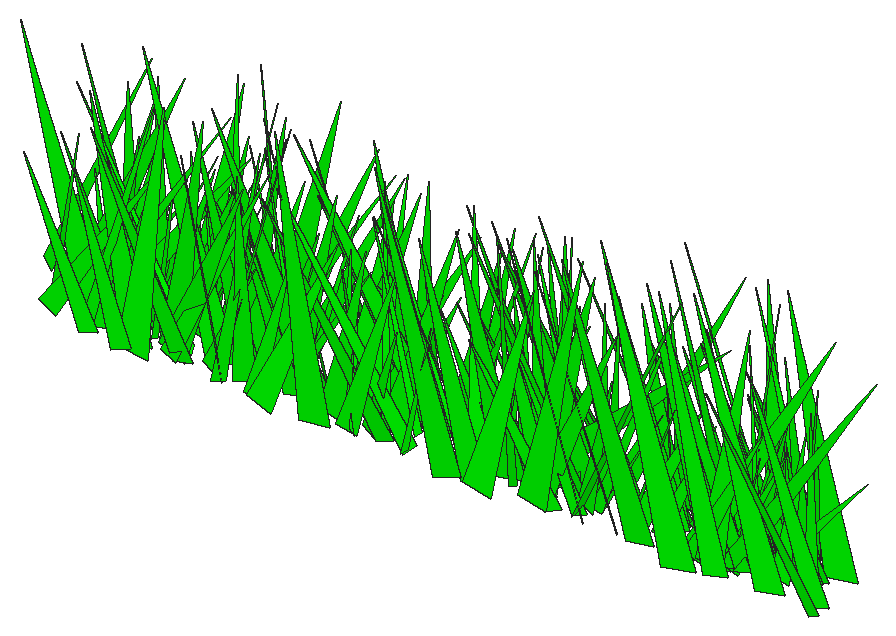
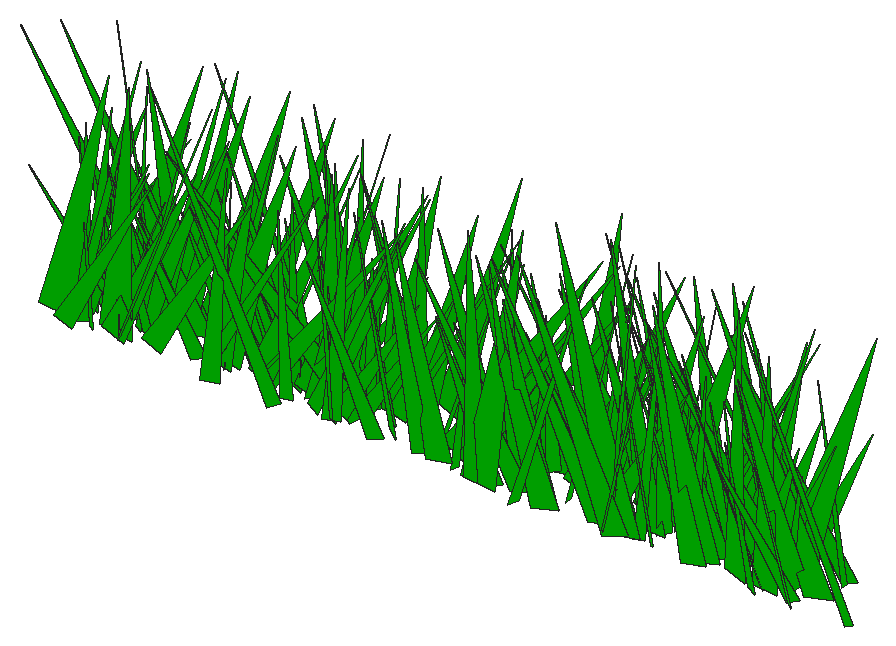
# SketchUp Ruby script. Lengths in inches.
U = 1.inch
M = Sketchup.active_model
def pt(a) = Geom::Point3d.new(a.map { |v| v * U })
def face(e, loops, mat)
  f = e.add_face(loops[0].map { |a| pt(a) })
  loops[1..].each { |l| e.add_face(l.map { |a| pt(a) }).erase! }
  f.material = f.back_material = mat if mat
  f
end
# faces: each face lists its corners as indices into pts; further lists are holes
def faces(e, pts, list, mat = nil) = list.each { |f| face(e, (f[0].is_a?(Array) ? f : [f]).map { |l| l.map { |i| pts[i] } }, mat) }
# xy, xz, yz: faces in a plane at the given z, y or x. An outline is a flat list of corners, or four numbers for a rectangle; further outlines are holes
def ring(l) = l.size == 4 ? [[l[0], l[1]], [l[2], l[1]], [l[2], l[3]], [l[0], l[3]]] : l.each_slice(2).to_a
def flat(e, list, mat, &to3) = list.each { |f| face(e, (f[0].is_a?(Array) ? f : [f]).map { |l| ring(l).map { |u, v| to3.(u, v) } }, mat) }
def xy(e, z, list, mat = nil) = flat(e, list, mat) { |x, y| [x, y, z] }
def xz(e, y, list, mat = nil) = flat(e, list, mat) { |x, z| [x, y, z] }
def yz(e, x, list, mat = nil) = flat(e, list, mat) { |y, z| [x, y, z] }
def lines(e, pts, list) = list.each { |a, b| e.add_line(pt(pts[a]), pt(pts[b])) }
# prism: a flat outline (further loops are holes) pulled along v
def prism(e, loops, v, mat = nil)
  f = face(e, loops, mat); d = Geom::Vector3d.new(v.map { |x| x * U })
  f.pushpull(f.normal.samedirection?(d) ? d.length : -d.length)
end
def box(e, o, s, mat = nil) = prism(e, [[o, [o[0] + s[0], o[1], o[2]], [o[0] + s[0], o[1] + s[1], o[2]], [o[0], o[1] + s[1], o[2]]]], [0, 0, s[2]], mat)
def at(x, y, z, deg = 0) = Geom::Transformation.translation(pt([x, y, z])) * Geom::Transformation.rotation(ORIGIN, Z_AXIS, deg.degrees)
def axes(o, x, y, z) = Geom::Transformation.new([*x, 0, *y, 0, *z, 0, *pt(o).to_a, 1])
def part(name) = M.definitions.add(name)
# library, detail: a bought-in or finely detailed component or shape, given as its bounding box
def library(name, o, s) = part(name).tap { |d| box(d.entities, o, s) }
def detail(e, o, s) = box(e.add_group.entities, o, s)
def put(e, d, t, mat = nil) = e.add_instance(d, t).tap { |i| i.material = mat if mat }
def group(e, t, mat = nil) = e.add_group.tap { |g| g.transformation = t; g.material = mat if mat }.entities
root = M.entities
M.materials.add("[0065_Lime]").color = [0, 255, 0]
c1 = part("fur_instance\#9")
p = [[0.8125,0,1.79],[0.67,-0.02,1.48],[0,-0.11,0],[0,0.11,0]]
faces(c1.entities,p,[[0,1,2,3]])
put(root,c1,axes([102.21,26.05,1.48],[1.7547,1.16122,2.32218],[-8.46058,0.32869,-1.27782],[-2.20466,-0.33717,6.75196]),"[0065_Lime]")
put(root,c1,axes([123.31,25.84,1.48],[-1.5424,1.29726,0.5634],[-9.04708,-0.19027,-1.70729],[-1.96466,-0.14229,7.41961]),"[0065_Lime]")
put(root,c1,axes([111.69,25.86,1.48],[-1.10332,1.04471,0.27422],[-7.18185,-0.16201,1.56413],[1.95185,-0.00559,5.91025]),"[0065_Lime]")
put(root,c1,axes([109.89,25.96,1.48],[3.37414,1.16063,2.27988],[-7.67588,0.59567,-2.64497],[-4.14231,-0.15841,6.75834]),"[0065_Lime]")
put(root,c1,axes([106.98,26.59,1.48],[4.6883,-0.22426,0.48877],[1.33627,0.63657,1.30663],[-1.05954,-0.18951,3.81064]),"[0065_Lime]")
put(root,c1,axes([91.18,25.96,1.48],[1.11734,0.80378,0.05922],[-5.21364,0.14737,-1.94062],[-2.35444,0.05511,4.32539]),"[0065_Lime]")
put(root,c1,axes([99.17,25.87,1.48],[-1.68486,0.94414,0.02379],[-6.07569,-0.21589,2.40069],[2.86921,0.09727,5.09755]),"[0065_Lime]")
put(root,c1,axes([91.78,26.04,1.48],[-1.91905,1.11623,1.28489],[-7.93462,-0.30486,1.0337],[1.62457,-0.17042,6.56651]),"[0065_Lime]")
put(root,c1,axes([98.54,26.24,1.48],[-1.07859,0.61607,1.11572],[-4.32863,-0.20259,0.97977],[1.53823,-0.13812,3.53945]),"[0065_Lime]")
put(root,c1,axes([130.69,26.3125,1.48],[-5.79002,-0.44025,0.10676],[3.0058,-0.76816,1.71372],[-0.89348,0.26874,5.07335]),"[0065_Lime]")
put(root,c1,axes([124.97,26.41,1.48],[-6.3055,0.74654,2.04882],[-5.78447,-0.88065,-1.02622],[1.05354,-0.36713,6.62786]),"[0065_Lime]")
put(root,c1,axes([89.08,26.29,1.48],[-2.14765,0.68234,0.54136],[-4.74981,-0.26455,-1.29382],[-1.20923,-0.17271,4.12059]),"[0065_Lime]")
put(root,c1,axes([114.36,26.49,1.48],[3.62527,0.99891,2.4784],[-7.73426,0.46872,1.15493],[-0.00819,-0.47235,6.38732]),"[0065_Lime]")
put(root,c1,axes([96.35,26.7,1.48],[-6.74477,-0.19585,1.4121],[1.05256,-0.96631,-1.16464],[1.96177,-0.1549,5.4798]),"[0065_Lime]")
put(root,c1,axes([111.2,26.3,1.48],[0.41444,0.99584,1.54491],[-7.02435,0.13106,-1.58405],[-2.11909,-0.23967,5.55294]),"[0065_Lime]")
put(root,c1,axes([103.67,26.52,1.48],[2.05749,-0.71511,1.47796],[5.3628,0.23665,-1.10273],[0.66397,0.30458,4.32675]),"[0065_Lime]")
put(root,c1,axes([116.95,26.78,1.48],[-8.41983,-0.27343,1.12929],[1.68169,-1.18523,-1.32039],[1.6988,-0.18194,6.9042]),"[0065_Lime]")
put(root,c1,axes([120.48,26.59,1.48],[-3.81513,-1.0233,1.83212],[7.58861,-0.4764,1.53917],[-0.72074,0.40077,6.5077]),"[0065_Lime]")
put(root,c1,axes([107.1,26.82,1.48],[-7.50723,0.41992,0.59815],[-3.0118,-0.94646,-2.74542],[-0.63269,-0.47719,5.97164]),"[0065_Lime]")
put(root,c1,axes([115.54,26.54,1.48],[-2.49387,0.61789,0.35428],[-4.10879,-0.29841,-1.697],[-1.62573,-0.19365,3.74544]),"[0065_Lime]")
put(root,c1,axes([104.59,27.01,1.48],[-2.3394,-0.59166,0.20628],[3.54462,-0.29782,-2.02693],[2.28668,-0.14364,3.35302]),"[0065_Lime]")
put(root,c1,axes([116.53,27.02,1.48],[9.28519,-0.22692,0.14299],[1.53138,1.27057,1.77261],[-0.54197,-0.29762,7.45832]),"[0065_Lime]")
put(root,c1,axes([94.07,26.78,1.48],[-4.00819,-0.79191,0.76199],[5.61604,-0.51668,1.55272],[-1.04793,0.25999,5.40673]),"[0065_Lime]")
put(root,c1,axes([93.17,27.14,1.48],[-1.34104,-1.06333,0.3975],[6.82997,-0.19967,-2.65233],[3.29441,-0.01889,5.6606]),"[0065_Lime]")
put(root,c1,axes([105.66,26.82,1.48],[-4.89101,-0.7549,0.09144],[5.11683,-0.64778,1.88363],[-1.64083,0.23016,5.60141]),"[0065_Lime]")
put(root,c1,axes([119.13,26.63,1.48],[-7.69959,-0.10862,0.71828],[0.9253,-1.0684,1.14867],[0.72189,0.21091,6.18874]),"[0065_Lime]")
put(root,c1,axes([111.54,26.7,1.48],[-7.68571,-0.19114,0.0547],[1.35022,-1.06232,1.1351],[-0.17805,0.19472,6.24652]),"[0065_Lime]")
put(root,c1,axes([114.32,27.02,1.48],[3.75349,-0.83573,0.21049],[5.86726,0.51206,-1.09875],[1.00756,0.13155,5.61414]),"[0065_Lime]")
put(root,c1,axes([97.33,27.16,1.48],[4.32558,-0.81356,0.76166],[5.55616,0.62078,1.34166],[-1.87806,-0.03725,5.72352]),"[0065_Lime]")
put(root,c1,axes([104.02,26.51,1.48],[4.22809,0.04304,1.71651],[0.74399,0.58735,-1.70596],[-1.99837,0.30972,2.99662]),"[0065_Lime]")
put(root,c1,axes([88.56,26.74,1.48],[7.61975,-0.23734,1.45771],[2.02283,1.07025,-1.15684],[-1.40453,0.25377,6.24217]),"[0065_Lime]")
put(root,c1,axes([93.22,26.82,1.48],[5.99973,0.64849,0.4783],[-4.63193,0.82003,1.18719],[0.43521,-0.21248,6.04147]),"[0065_Lime]")
put(root,c1,axes([127.85,26.72,1.48],[2.99159,-0.87631,4.59081],[7.42678,0.67032,1.08546],[-3.94812,0.59694,5.52044]),"[0065_Lime]")
put(root,c1,axes([114.21,27.2,1.48],[3.02124,-1.08196,0.95783],[7.76367,0.40389,-0.91484],[0.63141,0.21091,6.66551]),"[0065_Lime]")
put(root,c1,axes([102.27,27.125,1.48],[-0.14869,-0.83482,1.14694],[5.953,-0.06392,-1.04827],[1.35853,0.1887,4.71898]),"[0065_Lime]")
put(root,c1,axes([86.19,26.92,1.48],[4.36671,0.71514,0.39873],[-4.84361,0.54959,2.0661],[1.63745,-0.28142,5.04826]),"[0065_Lime]")
put(root,c1,axes([91.52,26.67,1.48],[-1.20291,1.07757,0.71265],[-7.6214,-0.14613,-1.10764],[-1.22014,-0.14958,6.21607]),"[0065_Lime]")
put(root,c1,axes([96.39,26.48,1.48],[6.48375,0.70369,0.55989],[-4.60974,0.88766,-2.06362],[-2.07422,0.22691,6.33633]),"[0065_Lime]")
put(root,c1,axes([130.41,26.98,1.48],[-4.31695,0.71055,1.29643],[-5.29641,-0.56479,-1.29621],[-0.24161,-0.31487,5.25057]),"[0065_Lime]")
put(root,c1,axes([116.68,26.99,1.48],[-3.03929,0.52441,0.66866],[-3.75819,-0.38343,-1.22573],[-0.69236,-0.22071,3.71813]),"[0065_Lime]")
put(root,c1,axes([86.16,27.32,1.48],[5.92393,0.15481,1.78214],[-1.86022,0.80815,1.7389],[-1.59798,-0.36688,4.58238]),"[0065_Lime]")
put(root,c1,axes([112.17,27.6,1.48],[1.49735,-1.20236,0.06671],[8.3405,0.20769,1.56803],[-1.91273,-0.03563,6.88965]),"[0065_Lime]")
put(root,c1,axes([123.05,27.09,1.48],[2.02452,-0.64693,1.18017],[4.62597,0.19687,-1.63434],[1.37886,0.28937,3.75031]),"[0065_Lime]")
put(root,c1,axes([96.22,26.6,1.48],[8.82311,0.3951,1.03383],[-2.25651,1.19516,-2.5638],[-2.10468,0.37495,7.08272]),"[0065_Lime]")
put(root,c1,axes([95.14,27.22,1.48],[3.25571,0.32358,0.89348],[-2.54741,0.39839,1.30694],[0.14161,-0.27277,2.96877]),"[0065_Lime]")
put(root,c1,axes([119.39,26.97,1.48],[5.10806,0.03443,0.5675],[-0.08817,0.70776,-0.91388],[-0.73419,0.15457,4.05811]),"[0065_Lime]")
put(root,c1,axes([124.47,27.18,1.48],[-2.0294,1.06878,2.47195],[-8.07706,-0.18812,-1.66187],[-1.35942,-0.47779,6.18385]),"[0065_Lime]")
put(root,c1,axes([125.18,27.48,1.48],[4.46412,-0.18338,0.40179],[1.0179,0.58709,1.49617],[-0.95449,-0.23159,3.47473]),"[0065_Lime]")
put(root,c1,axes([124.1,27.05,1.48],[4.86592,-0.74135,2.94554],[6.30982,0.66225,-1.31143],[-1.06488,0.53652,5.6888]),"[0065_Lime]")
put(root,c1,axes([92.95,27.55,1.48],[-2.67145,-1.06307,1.53834],[7.41878,-0.43302,-1.50304],[2.40291,0.15503,6.35076]),"[0065_Lime]")
put(root,c1,axes([89.19,26.93,1.48],[-1.2719,1.30197,0.61878],[-9.00315,-0.1456,-1.9784],[-2.31768,-0.14889,7.34561]),"[0065_Lime]")
put(root,c1,axes([126.86,27.16,1.48],[-6.89711,0.19534,2.04472],[-1.04841,-1.02654,0.94629],[2.67436,0.10134,5.64424]),"[0065_Lime]")
put(root,c1,axes([99.89,27.5,1.48],[-0.65863,-0.72216,0.74708],[5.05605,-0.05582,1.14126],[-1.30097,0.14868,4.05712]),"[0065_Lime]")
put(root,c1,axes([114.41,27.92,1.48],[7.30262,-0.46788,0.93542],[2.47118,0.94547,3.08221],[-2.51048,-0.43032,5.75496]),"[0065_Lime]")
put(root,c1,axes([103.85,27.76,1.48],[-4.5948,-0.46783,0.32278],[2.92083,-0.60494,-1.87066],[1.64644,-0.23241,4.2194]),"[0065_Lime]")
put(root,c1,axes([116.51,27.64,1.48],[-2.36556,-0.63281,0.7363],[4.04229,-0.35473,-1.6233],[2.1817,-0.02888,3.80603]),"[0065_Lime]")
put(root,c1,axes([124.99,27.3,1.48],[7.74588,-0.59537,0.16584],[4.07919,1.02912,-2.25937],[1.16355,0.35557,6.81694]),"[0065_Lime]")
put(root,c1,axes([112.71,27.1875,1.48],[-6.89012,-0.28564,2.5667],[2.88207,-0.99639,1.4033],[2.40473,0.37575,5.67232]),"[0065_Lime]")
put(root,c1,axes([125.5,27.34,1.48],[-0.53049,0.95921,1.54038],[-6.75326,0.01211,-1.79154],[-2.1394,-0.27608,5.27326]),"[0065_Lime]")
put(root,c1,axes([122.91,27.48,1.48],[6.46797,0.95534,0.6255],[-6.66624,0.84641,2.29021],[1.54112,-0.34829,7.28128]),"[0065_Lime]")
put(root,c1,axes([93.75,27.89,1.48],[-8.32403,-0.05832,0.19902],[0.34032,-1.13292,-1.70662],[0.34102,-0.29292,6.56096]),"[0065_Lime]")
put(root,c1,axes([89.32,27.81,1.48],[-2.17451,-0.51292,1.01396],[3.23893,-0.352,-1.37089],[2.09456,0.01183,3.17253]),"[0065_Lime]")
put(root,c1,axes([102.88,27.31,1.48],[-4.25924,0.50107,0.83309],[-3.18038,-0.60594,1.45415],[1.91047,0.10839,4.27804]),"[0065_Lime]")
put(root,c1,axes([125.24,27.78,1.48],[8.69972,0.19536,2.29007],[-1.9059,1.25464,1.20397],[-2.49537,-0.27716,7.0644]),"[0065_Lime]")
put(root,c1,axes([124.11,27.53,1.48],[1.86662,0.51381,0.05793],[-3.25481,0.22827,1.5491],[1.66779,-0.12959,2.95836]),"[0065_Lime]")
put(root,c1,axes([116.28,27.75,1.48],[-5.84124,-0.79171,0.3489],[5.57846,-0.79419,1.40547],[-0.89958,0.21588,6.45006]),"[0065_Lime]")
put(root,c1,axes([114.51,27.3125,1.48],[1.08248,0.8859,0.66112],[-5.90791,0.18297,-1.81537],[-2.34619,-0.05199,4.87629]),"[0065_Lime]")
put(root,c1,axes([124.61,27.59,1.48],[3.99779,-0.30536,0.53471],[2.26734,0.52734,-1.12481],[0.11703,0.21452,3.52618]),"[0065_Lime]")
put(root,c1,axes([111.54,27.71,1.48],[-0.31973,-0.63903,1.38287],[4.54843,0.04431,1.38188],[-1.69804,0.23901,3.44117]),"[0065_Lime]")
put(root,c1,axes([121.23,28,1.48],[-6.67326,-0.56344,0.77715],[3.79648,-0.93964,-1.25864],[1.60555,-0.12001,6.20631]),"[0065_Lime]")
put(root,c1,axes([113.48,28.23,1.48],[7.47731,-0.69771,1.27459],[4.16995,1.03321,2.76634],[-3.11784,-0.29141,6.75662]),"[0065_Lime]")
put(root,c1,axes([89.72,27.38,1.48],[-1.66786,1.00688,0.93672],[-6.96181,-0.26888,1.483],[2.05026,-0.0939,5.79765]),"[0065_Lime]")
put(root,c1,axes([117.22,27.96,1.48],[4.80949,0.02524,0.08041],[-0.20451,0.61412,1.63311],[-0.01483,-0.28246,3.55793]),"[0065_Lime]")
put(root,c1,axes([119.09,27.39,1.48],[-6.37147,0.18899,0.31836],[-1.12653,-0.84357,1.86359],[0.83252,0.30493,4.95819]),"[0065_Lime]")
put(root,c1,axes([129.65,27.43,1.48],[3.6883,0.6764,0.76546],[-4.49067,0.53223,-1.44316],[-1.97249,0.05307,4.71688]),"[0065_Lime]")
put(root,c1,axes([100.97,27.83,1.48],[-1.78592,-1.12756,2.19173],[8.08327,-0.11234,2.42134],[-2.51212,0.44013,6.233]),"[0065_Lime]")
put(root,c1,axes([125.47,28.19,1.48],[-1.32221,-0.82201,0.14414],[5.44298,-0.18209,-1.7626],[2.15095,-0.04451,4.54886]),"[0065_Lime]")
put(root,c1,axes([117.05,27.76,1.48],[6.43038,-0.27488,0.84573],[2.12393,0.89247,-0.96489],[-0.62976,0.20322,5.38141]),"[0065_Lime]")
put(root,c1,axes([97.4,27.5625,1.48],[2.91018,0.95681,1.90084],[-6.32064,0.50914,-2.18513],[-3.44613,-0.12582,5.61302]),"[0065_Lime]")
put(root,c1,axes([120.71,27.7,1.48],[1.31586,0.60821,0.09417],[-4.20499,0.17545,0.90538],[1.03265,-0.06059,3.56674]),"[0065_Lime]")
put(root,c1,axes([87.57,28.06,1.48],[8.70579,0.41849,0.09302],[-2.87223,1.1648,2.25868],[0.7957,-0.37417,7.13535]),"[0065_Lime]")
put(root,c1,axes([110.54,27.37,1.48],[-7.28352,0.68305,1.02357],[-4.22162,-1.0017,2.52328],[2.71851,0.2745,6.66084]),"[0065_Lime]")
put(root,c1,axes([91.77,27.69,1.48],[4.40027,0.3254,0.89832],[-1.98729,0.62716,-1.17167],[-1.62258,0.11431,3.87119]),"[0065_Lime]")
put(root,c1,axes([125.14,27.86,1.48],[-7.90259,-0.54636,1.90568],[4.34491,-1.10179,1.33626],[1.3148,0.35712,7.03827]),"[0065_Lime]")
put(root,c1,axes([104.99,27.77,1.48],[6.93439,-0.08862,2.99387],[1.52726,1.06272,-1.28638],[-3.40767,0.29595,5.51579]),"[0065_Lime]")
put(root,c1,axes([106.49,28.18,1.48],[-6.46226,0.10875,1.49099],[-1.16464,-0.91643,-1.1],[1.61321,-0.22598,5.17851]),"[0065_Lime]")
put(root,c1,axes([88.61,28.81,1.48],[-6.29236,-0.83425,0.73641],[4.20963,-0.7441,-4.44776],[4.2833,-0.49426,5.45307]),"[0065_Lime]")
put(root,c1,axes([98.03,28.25,1.48],[-0.80672,-0.78785,0.98574],[5.3495,-0.1654,-1.5332],[2.07066,0.12037,4.34503]),"[0065_Lime]")
put(root,c1,axes([100.125,27.82,1.48],[-7.22886,0.19165,1.30553],[-1.00364,-1.02225,1.35158],[1.85173,0.1941,5.82915]),"[0065_Lime]")
put(root,c1,axes([115.83,28.61,1.48],[2.62945,-1.14277,0.36379],[7.52794,0.36619,2.54529],[-3.10951,-0.07981,6.46964]),"[0065_Lime]")
put(root,c1,axes([95.51,27.85,1.48],[-4.72421,1.13778,0.96379],[-8.15943,-0.64026,-1.13504],[-0.62439,-0.2418,7.54035]),"[0065_Lime]")
put(root,c1,axes([113.27,27.9375,1.48],[1.06621,0.7964,0.76881],[-5.59789,0.17444,-0.91843],[-1.2958,-0.09827,4.60022]),"[0065_Lime]")
put(root,c1,axes([95.25,27.875,1.48],[-4.74295,0.26373,0.69877],[-1.45129,-0.64119,1.59148],[1.46775,0.21822,3.83169]),"[0065_Lime]")
put(root,c1,axes([99.2,28.08,1.48],[4.82612,-0.24812,0.22341],[1.75994,0.64068,-1.31132],[0.3098,0.22563,3.96913]),"[0065_Lime]")
put(root,c1,axes([119.26,27.93,1.48],[0.27004,0.7269,0.1574],[-4.82835,0.02555,1.52705],[1.86668,-0.03907,3.92708]),"[0065_Lime]")
put(root,c1,axes([127.44,27.91,1.48],[-2.25923,0.65622,0.42776],[-4.42057,-0.32457,1.23705],[1.595,0.02994,4.03441]),"[0065_Lime]")
put(root,c1,axes([99.1,28.4375,1.48],[0.43021,-0.97827,1.06554],[6.94449,0.02181,-1.18405],[1.39926,0.19251,5.54877]),"[0065_Lime]")
put(root,c1,axes([112.87,27.86,1.48],[-3.60638,0.63054,0.151],[-4.29658,-0.49414,1.24673],[1.30741,0.11539,4.51368]),"[0065_Lime]")
put(root,c1,axes([89.1875,28.45,1.48],[6.48925,0.21547,1.68072],[-2.14119,0.88902,1.65076],[-1.42689,-0.35415,5.16649]),"[0065_Lime]")
put(root,c1,axes([96.4375,28.08,1.48],[1.7678,0.92045,1.0881],[-6.60091,0.20945,1.15859],[1.06086,-0.23059,5.39584]),"[0065_Lime]")
put(root,c1,axes([94.91,27.875,1.48],[8.64757,0.40401,1.27347],[-2.45765,1.21163,-1.83859],[-2.16279,0.23857,7.18101]),"[0065_Lime]")
put(root,c1,axes([125.7,28.24,1.48],[-4.07602,0.68508,1.04212],[-5.02154,-0.53152,-1.28644],[-0.44187,-0.27918,5.00645]),"[0065_Lime]")
put(root,c1,axes([91.26,28.29,1.48],[-6.8004,-0.68343,1.5184],[5.15089,-0.94663,0.9862],[0.77962,0.29296,6.72877]),"[0065_Lime]")
put(root,c1,axes([91.45,28.34,1.48],[-2.92412,0.5885,2.71072],[-4.35164,-0.57207,1.05581],[3.11589,-0.24668,4.01842]),"[0065_Lime]")
put(root,c1,axes([99.24,28.77,1.48],[-6.03143,-0.28719,0.19005],[1.88074,-0.81105,-1.57684],[0.83335,-0.24813,4.93422]),"[0065_Lime]")
put(root,c1,axes([104.99,28.33,1.48],[1.87388,0.94439,1.47459],[-6.87313,0.20924,1.28863],[1.10252,-0.30074,5.52706]),"[0065_Lime]")
put(root,c1,axes([125.57,28.73,1.48],[-7.1729,-0.03907,1.51397],[-0.27399,-0.99793,-1.7218],[1.86185,-0.29737,5.57927]),"[0065_Lime]")
put(root,c1,axes([100.73,28.91,1.48],[-8.43183,-0.41084,1.13239],[2.39705,-1.15871,-2.27753],[2.17731,-0.31537,6.89266]),"[0065_Lime]")
put(root,c1,axes([115.12,28.32,1.48],[-7.33301,-0.55939,1.12117],[4.21083,-0.96147,2.14772],[-0.1277,0.41815,6.43826]),"[0065_Lime]")
put(root,c1,axes([88.53,28.37,1.48],[4.54875,0.89432,0.22643],[-5.88316,0.57128,2.58952],[2.44381,-0.28935,5.81249]),"[0065_Lime]")
put(root,c1,axes([128.74,28.67,1.48],[-1.66187,-0.75635,0.54641],[5.29837,-0.20519,1.14462],[-1.16219,0.14608,4.43693]),"[0065_Lime]")
put(root,c1,axes([108.28,28.67,1.48],[-7.26836,-0.01733,0.93529],[-0.06876,-1.01999,-0.98677],[1.15438,-0.16986,5.83011]),"[0065_Lime]")
put(root,c1,axes([95.97,28.89,1.48],[6.74479,-0.85355,0.6921],[5.9693,0.95431,0.94789],[-1.41028,-0.04286,7.32215]),"[0065_Lime]")
put(root,c1,axes([99.8,28.33,1.48],[6.17481,-0.09706,1.26621],[1.16514,0.8408,-1.59967],[-1.24209,0.30619,4.79416]),"[0065_Lime]")
put(root,c1,axes([107.51,28.61,1.48],[-6.14358,0.91283,0.97046],[-6.32079,-0.74614,-2.95742],[-1.91608,-0.46544,6.64438]),"[0065_Lime]")
put(root,c1,axes([92.43,28.77,1.48],[5.87022,0.08395,0.56591],[-0.78335,0.78836,1.45733],[-0.47681,-0.26163,4.57298]),"[0065_Lime]")
put(root,c1,axes([111.41,28.26,1.48],[3.66856,0.38839,0.26337],[-2.46355,0.48825,-1.423],[-1.29444,0.17151,3.45463]),"[0065_Lime]")
put(root,c1,axes([128.69,28.42,1.48],[-4.57486,-0.5867,2.71896],[5.22273,-0.62329,1.30751],[1.15305,0.49537,4.86544]),"[0065_Lime]")
put(root,c1,axes([92.125,28.85,1.48],[1.15419,-0.84191,0.70262],[5.83914,0.12225,-1.43771],[1.59651,0.16152,4.75039]),"[0065_Lime]")
put(root,c1,axes([126.31,28.68,1.48],[3.48749,0.46515,0.01035],[-2.91466,0.43025,1.86383],[1.56936,-0.23461,3.43855]),"[0065_Lime]")
put(root,c1,axes([127.88,28.31,1.48],[3.38303,0.41215,0.36315],[-2.33564,0.42864,-1.9053],[-1.8295,0.2149,3.10392]),"[0065_Lime]")
put(root,c1,axes([118.74,28.71,1.48],[-7.01382,-0.73105,1.04403],[5.3585,-0.95585,1.39042],[-0.01836,0.30036,6.96588]),"[0065_Lime]")
put(root,c1,axes([116.81,28.5,1.48],[4.59382,0.57845,1.4682],[-3.92734,0.69293,-1.01775],[-2.18631,-0.02932,4.91315]),"[0065_Lime]")
put(root,c1,axes([86.34,28.94,1.48],[5.75193,-0.99995,0.33854],[7.05259,0.78737,-1.35183],[1.03656,0.19168,7.31905]),"[0065_Lime]")
put(root,c1,axes([120.38,29.04,1.48],[5.56204,-0.00812,2.15355],[-1.02334,0.7916,1.84877],[-2.44246,-0.35016,4.12952]),"[0065_Lime]")
put(root,c1,axes([89.11,28.73,1.48],[-3.11396,-0.58269,0.94882],[4.26881,-0.3903,1.23769],[-0.57752,0.2569,4.03252]),"[0065_Lime]")
put(root,c1,axes([91.39,28.47,1.48],[4.66465,0.33981,0.72446],[-2.12962,0.65402,-1.20702],[-1.45122,0.1325,4.09989]),"[0065_Lime]")
put(root,c1,axes([92.35,28.5,1.48],[7.19761,0.1753,0.29169],[-1.14577,0.99143,-1.2592],[-0.60999,0.20618,5.80696]),"[0065_Lime]")
put(root,c1,axes([114.05,29.11,1.48],[7.91638,-0.17186,2.27565],[0.44154,1.14539,1.88232],[-3.02123,-0.28293,6.23787]),"[0065_Lime]")
put(root,c1,axes([108.46,28.96,1.48],[7.64859,0.31283,1.33565],[-2.57271,1.05375,1.47745],[-1.01677,-0.313,6.30897]),"[0065_Lime]")
put(root,c1,axes([122.38,28.73,1.48],[3.67462,-0.25569,0.6366],[1.98077,0.4742,-1.1828],[0.00115,0.23204,3.1186]),"[0065_Lime]")
put(root,c1,axes([129.04,28.91,1.48],[-3.57787,-0.59573,0.53553],[4.236,-0.4714,1.15327],[-0.68061,0.19775,4.36253]),"[0065_Lime]")
put(root,c1,axes([112.79,28.75,1.48],[-3.72317,-0.4617,0.80863],[3.29969,-0.42451,1.93024],[-0.94658,0.33617,3.54805]),"[0065_Lime]")
put(root,c1,axes([120.85,28.52,1.48],[-0.64567,1.22402,0.84363],[-8.45141,-0.04763,-1.96397],[-2.35111,-0.16493,6.8281]),"[0065_Lime]")
put(root,c1,axes([90.08,28.63,1.48],[0.0026,0.72553,0.31083],[-4.94462,0.01627,-1.24504],[-1.53501,-0.05117,4.01109]),"[0065_Lime]")
put(root,c1,axes([95.41,28.68,1.48],[7.74767,-0.28473,3.40267],[3.01343,1.17763,-1.23775],[-3.53896,0.37941,6.39534]),"[0065_Lime]")
put(root,c1,axes([114.76,28.47,1.48],[2.8184,1.10701,0.43176],[-7.70435,0.40289,-1.33936],[-1.72878,0.00924,6.67276]),"[0065_Lime]")
put(root,c1,axes([126.64,29.12,1.48],[-4.75127,-0.04225,0.51902],[0.10084,-0.64497,-1.14871],[0.69814,-0.19441,3.69818]),"[0065_Lime]")
put(root,c1,axes([128.78,29.07,1.48],[-8.55723,0.16348,1.76076],[-1.4797,-1.22258,-0.9543],[1.96209,-0.209,6.95948]),"[0065_Lime]")
put(root,c1,axes([113.74,29.09,1.48],[-2.38155,-0.60945,0.20327],[4.12832,-0.30501,1.35894],[-1.35307,0.14211,3.78845]),"[0065_Lime]")
put(root,c1,axes([103.7,28.83,1.48],[-0.26902,0.65359,0.97332],[-4.34539,-0.10484,1.56449],[2.0454,-0.13678,3.45172]),"[0065_Lime]")
put(root,c1,axes([121.73,29.17,1.48],[0.15948,-0.65248,0.54426],[4.07387,-0.02739,-1.89014],[2.32642,0.09269,3.27258]),"[0065_Lime]")
put(root,c1,axes([98.5,29,1.48],[-1.30899,0.69969,1.52556],[-4.91523,-0.05507,-1.94407],[-2.03773,-0.31663,3.70934]),"[0065_Lime]")
put(root,c1,axes([112.7,28.89,1.48],[5.88869,-0.84366,0.2666],[4.9163,0.63844,-4.14906],[3.46189,0.52841,5.43867]),"[0065_Lime]")
put(root,c1,axes([90.6,29.63,1.48],[7.34387,-0.70869,1.1005],[4.29059,1.00596,2.76311],[-2.9761,-0.29849,6.69914]),"[0065_Lime]")
put(root,c1,axes([120.75,28.98,1.48],[0.56598,0.89713,1.69866],[-6.54535,0.13986,-1.03225],[-1.51023,-0.26995,5.11037]),"[0065_Lime]")
put(root,c1,axes([115.56,28.74,1.48],[-6.59409,0.48193,0.296],[-3.24405,-0.90414,1.51138],[1.17099,0.20907,5.85387]),"[0065_Lime]")
put(root,c1,axes([106.36,29.1875,1.48],[-3.98456,-0.7732,0.63342],[5.26903,-0.48281,2.1814],[-1.76667,0.3039,5.0773]),"[0065_Lime]")
put(root,c1,axes([88.21,28.88,1.48],[-3.53466,0.37763,0.11039],[-2.54269,-0.47904,1.04385],[0.88048,0.13257,3.45764]),"[0065_Lime]")
put(root,c1,axes([92.78,29.21,1.48],[0.14781,-0.74278,1.77927],[5.54739,-0.0565,-1.09534],[1.39755,0.30284,4.1596]),"[0065_Lime]")
put(root,c1,axes([124.86,28.93,1.48],[4.51595,0.49241,0.34809],[-3.38108,0.63135,-0.90481],[-1.01547,0.08767,4.56064]),"[0065_Lime]")
put(root,c1,axes([117.98,29.33,1.48],[-3.03502,-0.47601,0.12799],[3.18186,-0.38945,1.38653],[-1.17298,0.1752,3.42997]),"[0065_Lime]")
put(root,c1,axes([96.46,29.3125,1.48],[7.55479,0.55777,0.01917],[-3.85617,1.02957,1.68223],[0.94169,-0.25875,6.73485]),"[0065_Lime]")
put(root,c1,axes([117.96,29.3125,1.48],[-6.28029,-0.64517,0.07313],[4.31012,-0.82073,2.27743],[-1.58479,0.32458,5.90403]),"[0065_Lime]")
put(root,c1,axes([127.95,29.68,1.48],[-2.18415,-0.59855,0.1388],[4.02303,-0.29831,-1.22061],[1.41008,-0.07601,3.69747]),"[0065_Lime]")
put(root,c1,axes([110.65,29.11,1.48],[6.57801,0.37542,1.21361],[-2.32877,0.93661,-1.35711],[-1.98517,0.14527,5.61341]),"[0065_Lime]")
put(root,c1,axes([124.17,29.56,1.48],[-3.39271,-0.75841,0.27941],[5.18337,-0.43974,1.64664],[-1.54302,0.19036,4.91712]),"[0065_Lime]")
put(root,c1,axes([116.39,29.6,1.48],[-3.84572,-0.57392,1.57185],[3.96564,-0.59962,-0.91679],[2.16559,0.07883,4.47016]),"[0065_Lime]")
put(root,c1,axes([106.54,29.8125,1.48],[-4.61739,-0.44692,0.63068],[2.68886,-0.62521,-1.82078],[1.86731,-0.20484,4.1814]),"[0065_Lime]")
put(root,c1,axes([96.02,29.74,1.48],[-5.58073,-0.56065,1.2336],[3.71978,-0.81085,-1.21452],[2.09348,-0.05383,5.4465]),"[0065_Lime]")
put(root,c1,axes([92.92,29.78,1.48],[5.05704,-0.46823,1.28391],[2.76236,0.73049,1.72795],[-2.44215,-0.1433,4.61316]),"[0065_Lime]")
put(root,c1,axes([92.89,29.77,1.48],[5.6277,-0.14878,0.05453],[0.97482,0.74521,1.56908],[-0.41874,-0.26476,4.38573]),"[0065_Lime]")
put(root,c1,axes([88.99,29.75,1.48],[6.82447,-0.01001,0.14381],[0.0112,0.90932,1.76956],[-0.19028,-0.30553,5.26183]),"[0065_Lime]")
put(root,c1,axes([107.53,29.73,1.48],[0.65156,-0.95924,0.81527],[6.77144,0.06176,-1.14574],[1.32388,0.15622,5.45903]),"[0065_Lime]")
put(root,c1,axes([88.77,29.82,1.48],[4.13898,-0.88733,0.95981],[6.18361,0.60376,1.06065],[-1.74094,0.03493,6.04921]),"[0065_Lime]")
put(root,c1,axes([113.61,29.84,1.48],[-5.13453,-0.79388,1.0763],[5.4165,-0.74479,-1.31182],[2.08113,-0.0202,6.06968]),"[0065_Lime]")
put(root,c1,axes([113.53,29.82,1.48],[5.73284,-0.19475,1.19895],[0.86916,0.79906,1.5995],[-1.82702,-0.23095,4.52301]),"[0065_Lime]")
put(root,c1,axes([114.92,29.51,1.48],[-6.93401,-0.43843,0.70783],[3.23567,-0.95102,1.23304],[0.15153,0.24469,6.06076]),"[0065_Lime]")
put(root,c1,axes([121.12,29.38,1.48],[-7.49926,-0.34215,0.40559],[2.45753,-0.98745,2.15139],[-0.37165,0.37458,6.04188]),"[0065_Lime]")
put(root,c1,axes([126.14,29.85,1.48],[2.15264,-0.84054,1.56858],[5.28531,0.39709,2.33118],[-3.40082,0.08509,4.61584]),"[0065_Lime]")
put(root,c1,axes([104.22,29.92,1.48],[-0.1868,-0.74307,0.09996],[4.80324,-0.03107,-1.79939],[2.21531,0.0047,3.90988]),"[0065_Lime]")
put(root,c1,axes([125.93,29.82,1.48],[-3.29019,-0.33763,1.17885],[2.11758,-0.50467,-0.933],[1.84105,-0.02291,3.1799]),"[0065_Lime]")
put(root,c1,axes([95.19,29.86,1.48],[7.18984,-0.01784,1.47365],[-0.15691,1.0295,0.92409],[-1.80933,-0.16016,5.77577]),"[0065_Lime]")
put(root,c1,axes([97.32,29.96,1.48],[4.03136,0.03227,1.7101],[-1.03923,0.58407,1.25159],[-1.84194,-0.2589,3.03667]),"[0065_Lime]")
put(root,c1,axes([87.67,28.89,1.48],[-6.44526,0.92872,0.11363],[-5.22686,-0.7327,4.50944],[4.04747,0.5327,6.00439]),"[0065_Lime]")
put(root,c1,axes([108.55,29.65,1.48],[5.45498,-0.55024,2.10552],[4.51561,0.76741,-1.02045],[-1.28174,0.36185,5.36583]),"[0065_Lime]")
put(root,c1,axes([127.28,29.97,1.48],[5.66645,-0.10164,1.53775],[0.28868,0.82219,1.11715],[-2.00344,-0.169,4.51027]),"[0065_Lime]")
put(root,c1,axes([96.78,29.96,1.48],[3.44004,-1.19672,1.65495],[8.72496,0.44259,-1.27535],[0.7382,0.34571,7.36154]),"[0065_Lime]")
put(root,c1,axes([92.66,30.04,1.48],[-0.99761,-0.96699,1.38221],[6.76442,-0.20193,-1.50355],[2.11817,0.18944,5.4526]),"[0065_Lime]")
put(root,c1,axes([102.91,29.66,1.48],[3.72306,0.84109,0.27966],[-5.80444,0.4914,1.60362],[1.50171,-0.18587,5.505]),"[0065_Lime]")
put(root,c1,axes([103.2,29.26,1.48],[-6.70314,0.65976,1.39749],[-3.52513,-0.91001,3.20883],[3.54548,0.34257,5.83253]),"[0065_Lime]")
put(root,c1,axes([104.89,30.23,1.48],[0.26424,-1.2337,0.80503],[8.74895,0.05594,0.97242],[-1.232,0.13263,7.07824]),"[0065_Lime]")
put(root,c1,axes([98.36,29.74,1.48],[4.98527,0.85412,0.66975],[-6.04397,0.65856,1.62354],[1.04669,-0.26536,6.18495]),"[0065_Lime]")
put(root,c1,axes([104.98,30.24,1.48],[5.25224,-0.85736,0.8935],[5.93431,0.75382,1.15759],[-1.79389,-0.01653,6.44541]),"[0065_Lime]")
put(root,c1,axes([87.04,29.87,1.48],[1.91481,0.53417,0.67988],[-3.50559,0.17981,1.79862],[1.69125,-0.23208,2.9584]),"[0065_Lime]")
put(root,c1,axes([129.59,29.63,1.48],[-2.67099,1.16072,1.14964],[-8.34837,-0.35035,-0.9803],[-0.73118,-0.23993,6.99318]),"[0065_Lime]")
put(root,c1,axes([89.14,30.25,1.48],[4.64575,-0.22764,0.21351],[1.33796,0.58949,1.79815],[-0.95033,-0.28288,3.57536]),"[0065_Lime]")
put(root,c1,axes([83.71,30.05,1.48],[8.08706,0.41106,0.84209],[-3.09655,1.09541,1.75798],[-0.2018,-0.33554,6.77076]),"[0065_Lime]")
put(root,c1,axes([111,29.93,1.48],[3.48431,-0.53358,0.73708],[3.85679,0.44406,-1.29103],[0.60453,0.24236,3.98825]),"[0065_Lime]")
put(root,c1,axes([86.99,30.23,1.48],[6.65249,-0.04353,0.79578],[-0.03733,0.89087,1.8393],[-1.02551,-0.31479,5.09527]),"[0065_Lime]")
put(root,c1,axes([97.74,30.18,1.48],[-6.58436,-0.06997,1.39511],[0.02897,-0.92469,-1.46366],[1.78572,-0.24301,5.16782]),"[0065_Lime]")
put(root,c1,axes([101.73,29.52,1.48],[-1.37886,0.96886,0.03964],[-6.72225,-0.19045,1.26482],[1.53412,0.0363,5.57785]),"[0065_Lime]")
put(root,c1,axes([125.79,29.76,1.48],[-9.16115,0.05151,0.80785],[-0.19729,-1.27748,1.24916],[1.0401,0.21138,7.3524]),"[0065_Lime]")
put(root,c1,axes([101.05,30.22,1.48],[0.99495,-1.04398,1.054],[7.27947,0.08494,-1.72753],[1.97128,0.21327,5.84736]),"[0065_Lime]")
put(root,c1,axes([126.13,29.65,1.48],[1.90586,1.20364,0.99043],[-8.50021,0.29316,-1.11575],[-1.61298,-0.1227,7.05016]),"[0065_Lime]")
put(root,c1,axes([97.6,29.91,1.48],[-8.43042,-0.19864,2.53864],[1.93242,-1.23753,1.0011],[2.82925,0.25334,6.88071]),"[0065_Lime]")
put(root,c1,axes([102.51,30.65,1.48],[-7.89334,-0.56471,0.21523],[3.61983,-1.0306,-2.774],[1.76562,-0.41167,6.64938]),"[0065_Lime]")
put(root,c1,axes([92.35,29.62,1.48],[-2.81956,1.15408,0.85666],[-7.8813,-0.42199,1.88677],[2.5395,-0.02827,6.80668]),"[0065_Lime]")
put(root,c1,axes([120.07,30.49,1.48],[-4.08602,-0.84213,0.52566],[5.79407,-0.57897,-1.28161],[1.66232,-0.05198,5.75917]),"[0065_Lime]")
put(root,c1,axes([116.46,30.39,1.48],[8.28357,0.59997,1.30632],[-4.54096,1.03985,3.04843],[0.43539,-0.56966,6.94042]),"[0065_Lime]")
put(root,c1,axes([97.0625,30.15,1.48],[5.25882,-0.86361,1.47176],[6.36555,0.66708,-1.93254],[0.72535,0.40707,6.28928]),"[0065_Lime]")
put(root,c1,axes([128.63,30.32,1.48],[-2.82693,-0.74172,0.42805],[5.10369,-0.35746,1.54584],[-1.44616,0.18838,4.61872]),"[0065_Lime]")
